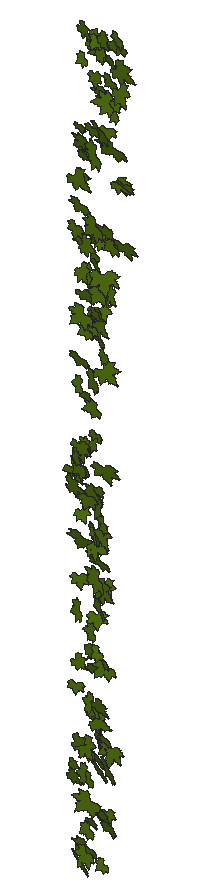
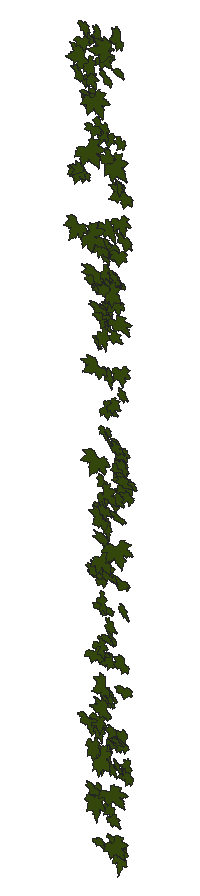
# SketchUp Ruby script. Lengths in inches.
U = 1.inch
M = Sketchup.active_model
def pt(a) = Geom::Point3d.new(a.map { |v| v * U })
def face(e, loops, mat)
  f = e.add_face(loops[0].map { |a| pt(a) })
  loops[1..].each { |l| e.add_face(l.map { |a| pt(a) }).erase! }
  f.material = f.back_material = mat if mat
  f
end
# faces: each face lists its corners as indices into pts; further lists are holes
def faces(e, pts, list, mat = nil) = list.each { |f| face(e, (f[0].is_a?(Array) ? f : [f]).map { |l| l.map { |i| pts[i] } }, mat) }
# xy, xz, yz: faces in a plane at the given z, y or x. An outline is a flat list of corners, or four numbers for a rectangle; further outlines are holes
def ring(l) = l.size == 4 ? [[l[0], l[1]], [l[2], l[1]], [l[2], l[3]], [l[0], l[3]]] : l.each_slice(2).to_a
def flat(e, list, mat, &to3) = list.each { |f| face(e, (f[0].is_a?(Array) ? f : [f]).map { |l| ring(l).map { |u, v| to3.(u, v) } }, mat) }
def xy(e, z, list, mat = nil) = flat(e, list, mat) { |x, y| [x, y, z] }
def xz(e, y, list, mat = nil) = flat(e, list, mat) { |x, z| [x, y, z] }
def yz(e, x, list, mat = nil) = flat(e, list, mat) { |y, z| [x, y, z] }
def lines(e, pts, list) = list.each { |a, b| e.add_line(pt(pts[a]), pt(pts[b])) }
# prism: a flat outline (further loops are holes) pulled along v
def prism(e, loops, v, mat = nil)
  f = face(e, loops, mat); d = Geom::Vector3d.new(v.map { |x| x * U })
  f.pushpull(f.normal.samedirection?(d) ? d.length : -d.length)
end
def box(e, o, s, mat = nil) = prism(e, [[o, [o[0] + s[0], o[1], o[2]], [o[0] + s[0], o[1] + s[1], o[2]], [o[0], o[1] + s[1], o[2]]]], [0, 0, s[2]], mat)
def at(x, y, z, deg = 0) = Geom::Transformation.translation(pt([x, y, z])) * Geom::Transformation.rotation(ORIGIN, Z_AXIS, deg.degrees)
def axes(o, x, y, z) = Geom::Transformation.new([*x, 0, *y, 0, *z, 0, *pt(o).to_a, 1])
def part(name) = M.definitions.add(name)
# library, detail: a bought-in or finely detailed component or shape, given as its bounding box
def library(name, o, s) = part(name).tap { |d| box(d.entities, o, s) }
def detail(e, o, s) = box(e.add_group.entities, o, s)
def put(e, d, t, mat = nil) = e.add_instance(d, t).tap { |i| i.material = mat if mat }
def group(e, t, mat = nil) = e.add_group.tap { |g| g.transformation = t; g.material = mat if mat }.entities
root = M.entities
M.materials.add("[Vegetation Blur 03]").color = [83, 114, 18]
c1 = part("ivy")
xy(c1.entities,0,[[0.782,0,0.786,0,0.787,0.005,0.789,0.009,0.821,0.072,0.875,0.147,1.001,0.272,1.073,0.331,1.137,0.363,1.178,0.379,1.223,0.384,1.272,0.383,1.311,0.374,1.36,0.355,1.399,0.334,1.491,0.285,1.541,0.244,1.583,0.199,1.617,0.15,1.64,0.128,1.662,0.115,1.717,0.105,1.745,0.093,1.784,0.054,1.819,0.057,1.854,0.064,1.882,0.075,1.896,0.074,1.91,0.071,1.937,0.063,1.964,0.053,1.99,0.038,2.016,0.015,2.034,0.002,2.04,0,2.038,0.003,2.036,0.007,2.033,0.038,2.036,0.068,2.045,0.1,2.055,0.116,2.064,0.123,2.077,0.129,2.088,0.129,2.106,0.132,2.118,0.13,2.179,0.132,2.207,0.133,2.225,0.133,2.242,0.138,2.22,0.162,2.207,0.186,2.206,0.213,2.212,0.236,2.228,0.262,2.247,0.274,2.298,0.283,2.355,0.294,2.37,0.296,2.376,0.295,2.377,0.3,2.377,0.303,2.385,0.329,2.411,0.37,2.426,0.392,2.449,0.407,2.511,0.426,2.561,0.444,2.619,0.466,2.589,0.469,2.561,0.476,2.501,0.5,2.449,0.516,2.424,0.523,2.401,0.535,2.377,0.556,2.372,0.568,2.36,0.575,2.268,0.586,2.225,0.592,2.207,0.599,2.194,0.61,2.143,0.65,2.13,0.664,2.122,0.682,2.123,0.7,2.13,0.719,2.148,0.75,2.17,0.781,2.195,0.807,2.221,0.828,2.284,0.874,2.291,0.88,2.288,0.887,2.276,0.9,2.267,0.916,2.265,0.933,2.273,0.967,2.292,1.002,2.313,1.03,2.334,1.054,2.348,1.067,2.358,1.074,2.363,1.076,2.362,1.081,2.35,1.094,2.347,1.11,2.35,1.143,2.359,1.18,2.385,1.254,2.415,1.324,2.448,1.393,2.45,1.4,2.446,1.398,2.44,1.394,2.427,1.383,2.402,1.36,2.376,1.339,2.345,1.324,2.305,1.309,2.282,1.303,2.273,1.306,2.245,1.294,2.212,1.287,2.187,1.291,2.163,1.301,2.142,1.316,2.134,1.327,2.124,1.325,2.09,1.292,2.053,1.259,2.014,1.234,1.973,1.215,1.954,1.21,1.931,1.208,1.909,1.212,1.893,1.22,1.879,1.233,1.872,1.248,1.867,1.281,1.864,1.319,1.821,1.258,1.773,1.197,1.726,1.141,1.698,1.121,1.679,1.116,1.666,1.117,1.647,1.122,1.632,1.129,1.62,1.141,1.617,1.154,1.617,1.219,1.621,1.254,1.623,1.268,1.623,1.281,1.618,1.314,1.606,1.346,1.603,1.375,1.607,1.403,1.603,1.467,1.599,1.499,1.605,1.525,1.614,1.552,1.629,1.577,1.635,1.589,1.629,1.587,1.618,1.582,1.596,1.566,1.581,1.556,1.568,1.552,1.557,1.55,1.545,1.553,1.531,1.562,1.522,1.572,1.504,1.591,1.486,1.611,1.474,1.631,1.457,1.666,1.455,1.684,1.457,1.698,1.452,1.715,1.444,1.728,1.424,1.754,1.419,1.772,1.423,1.786,1.434,1.819,1.444,1.848,1.446,1.855,1.44,1.861,1.43,1.867,1.386,1.904,1.349,1.948,1.326,1.973,1.31,1.995,1.288,2.048,1.284,2.153,1.287,2.254,1.284,2.255,1.282,2.253,1.278,2.247,1.274,2.237,1.266,2.216,1.226,2.125,1.208,2.076,1.184,2.033,1.155,1.984,1.135,1.942,1.111,1.899,1.083,1.861,1.053,1.85,1.059,1.83,1.061,1.809,1.056,1.79,1.049,1.767,1.04,1.749,1.018,1.733,0.994,1.726,0.942,1.734,0.95,1.6875,0.944,1.645,0.932,1.608,0.911,1.585,0.881,1.58,0.854,1.582,0.828,1.588,0.785,1.618,0.773,1.625,0.775,1.614,0.779,1.598,0.796,1.502,0.818,1.402,0.861,1.283,0.882,1.224,0.894,1.174,0.892,1.148,0.886,1.123,0.881,1.107,0.872,1.099,0.849,1.094,0.818,1.092,0.789,1.098,0.762,1.107,0.753,1.113,0.721,1.139,0.698,1.163,0.678,1.194,0.665,1.224,0.628,1.28,0.612,1.312,0.606,1.327,0.606,1.314,0.599,1.282,0.594,1.267,0.581,1.256,0.544,1.245,0.512,1.244,0.473,1.249,0.444,1.256,0.382,1.288,0.339,1.306,0.324,1.316,0.317,1.324,0.309,1.326,0.27,1.314,0.227,1.313,0.185,1.3125,0.152,1.317,0.122,1.328,0.092,1.345,0.073,1.353,0.079,1.338,0.092,1.308,0.117,1.249,0.13,1.215,0.139,1.164,0.147,1.148,0.157,1.136,0.163,1.122,0.174,1.086,0.177,1.067,0.182,1.054,0.186,1.043,0.191,1.038,0.211,1.028,0.237,1.005,0.25,0.974,0.253,0.96,0.25,0.944,0.242,0.914,0.243,0.906,0.249,0.902,0.26,0.894,0.289,0.88,0.307,0.873,0.322,0.862,0.364,0.799,0.403,0.738,0.431,0.709,0.439,0.691,0.441,0.678,0.4375,0.66,0.428,0.645,0.394,0.623,0.303,0.594,0.255,0.581,0.214,0.577,0.179,0.573,0.173,0.568,0.175,0.561,0.167,0.55,0.141,0.523,0.113,0.503,0.077,0.49,0.045,0.486,0.026,0.485,0.019,0.486,0.011,0.483,0,0.471,0.014,0.467,0.044,0.455,0.058,0.447,0.07,0.438,0.097,0.411,0.125,0.394,0.158,0.377,0.174,0.366,0.182,0.359,0.185,0.361,0.242,0.331,0.253,0.316,0.258,0.303,0.262,0.283,0.274,0.278,0.308,0.274,0.341,0.252,0.366,0.226,0.366,0.222,0.37,0.22,0.38,0.221,0.395,0.221,0.425,0.216,0.45,0.207,0.465,0.192,0.473,0.178,0.484,0.15,0.489,0.116,0.483,0.089,0.468,0.058,0.45,0.035,0.435,0.018,0.429,0.011,0.434,0.012,0.438,0.014,0.469,0.019,0.542,0.016,0.581,0.015,0.612,0.027,0.68,0.055,0.696,0.057,0.712,0.052,0.73,0.045,0.741,0.036,0.766,0.014]])
p = [[138.74,174.5,142.56],[138.66,174.5,142.56]]
lines(root,p,[[0,1]])
put(root,c1,axes([134.2,173.7,121.63],[0.07333,0.12212,0.31359],[0.38829,0.01811,-0.06159],[0.01986,-0.80476,0.0462]),"[Vegetation Blur 03]")
put(root,c1,axes([134.3,173.7,106.65],[0.09053,-0.05831,0.23092],[0.28382,-0.01925,-0.07488],[-0.01758,-0.61103,-0.01968]),"[Vegetation Blur 03]")
put(root,c1,axes([134.28,173.7,111.08],[0.35798,0.03491,0.00358],[0.00487,-0.0205,-0.29237],[0.01684,-0.73641,0.00831]),"[Vegetation Blur 03]")
put(root,c1,axes([134.47,173.7,128.12],[0.41941,-0.00434,-0.1684],[-0.2031,0.16133,-0.33757],[-0.03648,-0.94822,-0.05667]),"[Vegetation Blur 03]")
put(root,c1,axes([133.875,173.7,121.9],[0.48195,0.00963,0.21143],[0.25864,0.04977,-0.39304],[0.01557,-1.12486,-0.01558]),"[Vegetation Blur 03]")
put(root,c1,axes([134.5625,173.7,136.09],[0.40291,0.01111,-0.21009],[-0.25613,0.11786,-0.3262],[-0.02632,-0.9768,-0.04175]),"[Vegetation Blur 03]")
put(root,c1,axes([135.08,173.7,126.88],[0.08976,-0.09939,-0.28739],[-0.34963,0.10974,-0.07871],[-0.06393,-0.7397,0.02694]),"[Vegetation Blur 03]")
put(root,c1,axes([135.09,173.7,139.4],[0.2991,0.11532,-0.48246],[-0.59082,0.19391,-0.23668],[-0.05934,-1.34945,-0.07524]),"[Vegetation Blur 03]")
put(root,c1,axes([134.46,173.7,118.99],[0.56725,0.10726,-0.27566],[-0.34171,0.20149,-0.45603],[-0.00596,-1.34353,-0.0904]),"[Vegetation Blur 03]")
put(root,c1,axes([134.92,173.7,115.48],[0.25494,-0.21897,-0.29058],[-0.35433,0.12452,-0.22182],[-0.11199,-0.89248,0.04035]),"[Vegetation Blur 03]")
put(root,c1,axes([134.16,173.7,106.08],[0.21568,-0.13397,0.30172],[0.37321,-0.01782,-0.17894],[-0.04036,-0.88058,-0.04228]),"[Vegetation Blur 03]")
put(root,c1,axes([134.34,173.7,134.82],[0.45457,-0.14322,-0.01986],[-0.02603,-0.01905,-0.37516],[-0.06898,-0.93657,0.01067]),"[Vegetation Blur 03]")
put(root,c1,axes([134.97,173.7,103.27],[0.36107,0.086,-0.36328],[-0.44668,0.11955,-0.29126],[-0.01905,-1.17336,-0.0563]),"[Vegetation Blur 03]")
put(root,c1,axes([134.21,173.7,120.8],[0.10325,-0.14377,0.42811],[0.52829,-0.03594,-0.08677],[-0.03077,-1.09956,-0.05314]),"[Vegetation Blur 03]")
put(root,c1,axes([134.5,173.7,102.52],[0.54071,-0.2448,-0.19934],[-0.20803,0.34691,-0.44288],[-0.17473,-1.17061,-0.08956]),"[Vegetation Blur 03]")
put(root,c1,axes([134.57,173.7,134.13],[0.37713,0.02521,-0.05482],[-0.06814,0.09104,-0.30568],[0.00422,-0.78299,-0.03731]),"[Vegetation Blur 03]")
put(root,c1,axes([134.875,173.7,130.76],[0.44525,-0.05596,-0.30949],[-0.38019,-0.06333,-0.36251],[-0.0007,-1.20185,0.03351]),"[Vegetation Blur 03]")
put(root,c1,axes([135.45,173.7,132.39],[0.11247,0.10768,-0.41349],[-0.50254,0.19726,-0.08297],[-0.08291,-1.04957,-0.05801]),"[Vegetation Blur 03]")
put(root,c1,axes([134.4,173.7,116.58],[0.38704,0.02073,0.09682],[0.11906,-0.06304,-0.31489],[0.00062,-0.83064,0.02631]),"[Vegetation Blur 03]")
put(root,c1,axes([134.79,173.7,123.08],[0.46711,-0.27655,-0.25561],[-0.31156,0.09667,-0.39569],[-0.13813,-1.15324,0.02812]),"[Vegetation Blur 03]")
put(root,c1,axes([134.6,173.7,139.86],[0.29162,-0.09248,0.04712],[0.06325,0.07335,-0.23812],[-0.03677,-0.60733,-0.03593]),"[Vegetation Blur 03]")
put(root,c1,axes([134.36,173.7,111.95],[0.20869,-0.00294,0.30527],[0.37402,-0.00987,-0.17032],[-0.00489,-0.88135,0.00089]),"[Vegetation Blur 03]")
put(root,c1,axes([134.53,173.7,122.5625],[0.11578,-0.07742,0.31422],[0.36947,-0.22297,-0.09932],[-0.11465,-0.79672,-0.00274]),"[Vegetation Blur 03]")
put(root,c1,axes([134.08,173.7,136.79],[0.38841,-0.03974,0.39058],[0.47889,0.01108,-0.31703],[-0.00798,-1.26829,-0.01501]),"[Vegetation Blur 03]")
put(root,c1,axes([134.88,173.7,137.65],[0.29613,-0.07388,-0.10232],[-0.12287,0.05638,-0.24327],[-0.04369,-0.65932,-0.00934]),"[Vegetation Blur 03]")
put(root,c1,axes([135.37,173.7,107.11],[0.14128,-0.20319,-0.29587],[-0.36071,0.14973,-0.1309],[-0.10517,-0.78653,0.05152]),"[Vegetation Blur 03]")
put(root,c1,axes([135.1,173.7,143.71],[0.23115,-0.1069,-0.165],[-0.20647,-0.0259,-0.19002],[-0.03067,-0.63139,0.03573]),"[Vegetation Blur 03]")
put(root,c1,axes([135.41,173.7,126.21],[0.08326,0.10722,-0.24971],[-0.31037,0.02564,-0.0672],[0.00148,-0.65202,-0.0437]),"[Vegetation Blur 03]")
put(root,c1,axes([134.48,173.7,107.61],[0.11289,-0.08937,0.40816],[0.50197,0.01041,-0.09212],[-0.00461,-1.05497,-0.03549]),"[Vegetation Blur 03]")
put(root,c1,axes([135.47,173.7,123.94],[0.13432,-0.12713,-0.31462],[-0.38869,0.03529,-0.11278],[-0.03669,-0.83931,0.04291]),"[Vegetation Blur 03]")
put(root,c1,axes([134.91,173.7,138.74],[0.29319,-0.08212,-0.05398],[-0.06371,0.04494,-0.24127],[-0.04367,-0.61685,-0.01039]),"[Vegetation Blur 03]")
put(root,c1,axes([134.6,173.7,119.81],[0.27283,0.0757,0.1916],[0.23721,-0.13013,-0.2169],[-0.01401,-0.72914,0.0586]),"[Vegetation Blur 03]")
put(root,c1,axes([134.38,173.7,123.48],[0.52424,-0.12738,0.15619],[0.18843,-0.07357,-0.4307],[-0.07036,-1.14606,0.01029]),"[Vegetation Blur 03]")
put(root,c1,axes([135.38,173.7,129.78],[0.19574,-0.01438,-0.25163],[-0.30815,-0.03945,-0.1593],[0.01245,-0.75048,0.0132]),"[Vegetation Blur 03]")
put(root,c1,axes([135.15,173.7,105.83],[0.47968,0.02946,-0.35016],[-0.4281,-0.06549,-0.39149],[0.03188,-1.32271,0.01158]),"[Vegetation Blur 03]")
put(root,c1,axes([135.65,173.7,132.9],[0.09556,-0.13792,-0.34176],[-0.41905,0.10501,-0.08471],[-0.06516,-0.87761,0.04357]),"[Vegetation Blur 03]")
put(root,c1,axes([134.79,173.7,122.375],[0.34163,-0.14558,0.05444],[0.07406,0.06471,-0.28235],[-0.063,-0.71335,-0.03672]),"[Vegetation Blur 03]")
put(root,c1,axes([134.59,173.7,132.14],[0.2559,0.03571,0.2999],[0.36108,-0.20047,-0.20147],[-0.07032,-0.89939,0.05682]),"[Vegetation Blur 03]")
put(root,c1,axes([135.25,173.7,108.26],[0.31122,-0.06083,-0.21678],[-0.26689,-0.02709,-0.25402],[-0.01391,-0.84152,0.02385]),"[Vegetation Blur 03]")
put(root,c1,axes([135.4,173.7,104.21],[0.24157,-0.07416,-0.2538],[-0.31175,0.01688,-0.19842],[-0.02861,-0.81014,0.0191]),"[Vegetation Blur 03]")
put(root,c1,axes([134.6,173.7,131.19],[0.40086,-0.0573,0.17483],[0.21594,0.13183,-0.32299],[0.00594,-0.92596,-0.0568]),"[Vegetation Blur 03]")
put(root,c1,axes([134.9,173.7,138.23],[0.11718,-0.12684,0.22641],[0.28293,-0.00575,-0.09804],[-0.02661,-0.61967,-0.04543]),"[Vegetation Blur 03]")
put(root,c1,axes([134.81,173.7,121.18],[0.52679,-0.06661,-0.07919],[-0.09633,0.02908,-0.43069],[-0.03439,-1.10187,-0.00658]),"[Vegetation Blur 03]")
put(root,c1,axes([135.79,173.7,110.77],[0.05013,-0.17245,-0.31461],[-0.38087,0.18721,-0.05657],[-0.1028,-0.77773,0.05615]),"[Vegetation Blur 03]")
put(root,c1,axes([135,173.7,102.99],[0.48428,-0.17048,-0.13656],[-0.17611,-0.0992,-0.39652],[-0.06201,-1.04969,0.05965]),"[Vegetation Blur 03]")
put(root,c1,axes([135.89,173.7,107.78],[0.15704,0.2136,-0.46973],[-0.57168,0.3147,-0.1048],[-0.12334,-1.18664,-0.11235]),"[Vegetation Blur 03]")
put(root,c1,axes([135.49,173.7,106.8],[0.21308,-0.10262,-0.22404],[-0.27243,0.07685,-0.17812],[-0.0602,-0.71097,0.01308]),"[Vegetation Blur 03]")
put(root,c1,axes([135.8125,173.7,114.47],[0.09612,-0.08439,-0.33414],[-0.40558,0.12635,-0.08273],[-0.06933,-0.85613,0.02072]),"[Vegetation Blur 03]")
put(root,c1,axes([135.82,173.7,121.61],[0.20248,0.05039,-0.42079],[-0.51446,0.11243,-0.16277],[-0.042,-1.13431,-0.03483]),"[Vegetation Blur 03]")
put(root,c1,axes([134.9,173.7,133.32],[0.06821,0.02412,0.38984],[0.47536,-0.1037,-0.05439],[-0.04826,-0.98747,0.01524]),"[Vegetation Blur 03]")
put(root,c1,axes([134.76,173.7,144.75],[0.24867,-0.15858,0.33537],[0.40835,-0.11898,-0.21053],[-0.08971,-0.98119,-0.02867]),"[Vegetation Blur 03]")
put(root,c1,axes([135.82,173.7,125.97],[0.16222,0.03807,-0.33908],[-0.41557,-0.02093,-0.13279],[0.01621,-0.91758,-0.01104]),"[Vegetation Blur 03]")
put(root,c1,axes([134.57,173.7,107.83],[0.38921,-0.01895,0.37093],[0.44943,-0.16908,-0.31546],[-0.06835,-1.21968,0.03797]),"[Vegetation Blur 03]")
put(root,c1,axes([135.86,173.7,133.18],[0.08292,0.05054,-0.29306],[-0.34577,0.22171,-0.05915],[-0.09993,-0.72524,-0.0385]),"[Vegetation Blur 03]")
put(root,c1,axes([135.69,173.7,118.22],[0.33518,0.12814,-0.38098],[-0.46864,0.20726,-0.26366],[-0.04654,-1.16428,-0.08887]),"[Vegetation Blur 03]")
put(root,c1,axes([135.77,173.7,139.36],[0.33503,-0.17484,-0.44401],[-0.53885,0.1655,-0.28108],[-0.11328,-1.30432,0.02385]),"[Vegetation Blur 03]")
put(root,c1,axes([136.19,173.7,121.03],[0.10156,-0.07064,-0.4993],[-0.59327,0.30784,-0.08723],[-0.15326,-1.23847,0.0068]),"[Vegetation Blur 03]")
put(root,c1,axes([135.29,173.7,140.1],[0.37183,-0.05449,-0.06268],[-0.07386,0.08152,-0.30299],[-0.03383,-0.77703,-0.02739]),"[Vegetation Blur 03]")
put(root,c1,axes([135.92,173.7,117.5],[0.29364,-0.08887,-0.43973],[-0.53794,0.07502,-0.24166],[-0.05272,-1.26047,0.01662]),"[Vegetation Blur 03]")
put(root,c1,axes([135.3,173.7,109.67],[0.05383,0.00628,0.24765],[0.29967,-0.10102,-0.04299],[-0.04781,-0.62607,0.00942]),"[Vegetation Blur 03]")
put(root,c1,axes([135.78,173.7,134.52],[0.25146,0.10077,-0.27244],[-0.33679,0.12568,-0.19974],[-0.01997,-0.85077,-0.06178]),"[Vegetation Blur 03]")
put(root,c1,axes([135.6,173.7,135.57],[0.45075,-0.16208,-0.3284],[-0.40131,0.07789,-0.37294],[-0.08406,-1.24093,0.01948]),"[Vegetation Blur 03]")
put(root,c1,axes([135.22,173.7,111.97],[0.19108,-0.09038,0.20852],[0.25839,0.11931,-0.14958],[0.021,-0.6456,-0.05683]),"[Vegetation Blur 03]")
put(root,c1,axes([135.69,173.7,133.79],[0.23501,-0.07019,-0.1629],[-0.19555,0.08472,-0.19365],[-0.05258,-0.62881,-0.00791]),"[Vegetation Blur 03]")
put(root,c1,axes([135.2,173.7,113.14],[0.25479,-0.12423,0.18023],[0.21133,-0.13383,-0.2135],[-0.08804,-0.68079,0.00908]),"[Vegetation Blur 03]")
put(root,c1,axes([135.62,173.7,119.66],[0.37161,-0.21861,-0.25288],[-0.28876,0.23657,-0.31481],[-0.15463,-0.96714,-0.01984]),"[Vegetation Blur 03]")
put(root,c1,axes([135.25,173.7,104.28],[0.2775,-0.12673,0.11481],[0.14869,0.07236,-0.22682],[-0.03837,-0.63611,-0.04867]),"[Vegetation Blur 03]")
put(root,c1,axes([135.95,173.7,144.4],[0.21316,0.03069,-0.31446],[-0.38542,0.04396,-0.17335],[-0.01149,-0.90506,-0.01908]),"[Vegetation Blur 03]")
put(root,c1,axes([135.87,173.7,130.06],[0.16581,-0.12598,-0.20066],[-0.24842,0.03821,-0.1405],[-0.04988,-0.60905,0.03269]),"[Vegetation Blur 03]")
put(root,c1,axes([136.05,173.7,115.84],[0.20676,-0.07941,-0.38547],[-0.44776,0.31453,-0.17016],[-0.15519,-1.01328,-0.02261]),"[Vegetation Blur 03]")
put(root,c1,axes([135.78,173.7,129.8],[0.3273,-0.0909,-0.29956],[-0.34726,0.27044,-0.26563],[-0.12681,-0.97518,-0.04574]),"[Vegetation Blur 03]")
put(root,c1,axes([135.56,173.7,127.63],[0.43303,-0.27941,-0.22313],[-0.26455,0.14367,-0.37028],[-0.1523,-1.044,0.00876]),"[Vegetation Blur 03]")
put(root,c1,axes([135.47,173.7,107.71],[0.5589,-0.19272,-0.25961],[-0.28238,0.39595,-0.45114],[-0.17385,-1.26271,-0.10184]),"[Vegetation Blur 03]")
put(root,c1,axes([135.56,173.7,124.42],[0.33014,-0.06379,-0.05513],[-0.06679,0.02302,-0.2706],[-0.03261,-0.69306,-0.00391]),"[Vegetation Blur 03]")
put(root,c1,axes([135.44,173.7,109.71],[0.13106,0.04715,0.22271],[0.27208,-0.09295,-0.10355],[-0.03102,-0.61597,0.03267]),"[Vegetation Blur 03]")
put(root,c1,axes([135.42,173.7,130.65],[0.34203,-0.05341,0.04309],[0.05121,-0.04542,-0.27956],[-0.02898,-0.71072,0.01463]),"[Vegetation Blur 03]")
put(root,c1,axes([135.64,173.7,144.8125],[0.33694,0.0048,-0.1079],[-0.13035,-0.11296,-0.27192],[0.0222,-0.7362,0.04102]),"[Vegetation Blur 03]")
put(root,c1,axes([135.44,173.7,123.48],[0.09035,0.0602,0.28294],[0.33236,-0.23291,-0.06289],[-0.10289,-0.69949,0.04529]),"[Vegetation Blur 03]")
put(root,c1,axes([135.89,173.7,113.49],[0.26178,-0.07777,-0.19292],[-0.23918,-0.11506,-0.20887],[0.01,-0.71663,0.05447]),"[Vegetation Blur 03]")
put(root,c1,axes([135.35,173.7,114.91],[0.41222,0.08825,0.09854],[0.12607,-0.1297,-0.333],[0.02291,-0.87434,0.05934]),"[Vegetation Blur 03]")
put(root,c1,axes([135.25,173.7,117.91],[0.09143,0.21564,0.47102],[0.58317,-0.16267,-0.06368],[-0.06308,-1.19139,0.09395]),"[Vegetation Blur 03]")
put(root,c1,axes([135.94,173.7,113.27],[0.3587,-0.08547,-0.26789],[-0.31864,0.17898,-0.29317],[-0.08908,-0.98439,-0.03004]),"[Vegetation Blur 03]")
put(root,c1,axes([135.69,173.7,132.04],[0.46854,-0.05722,-0.15501],[-0.19159,-0.07548,-0.38134],[-0.0119,-1.03762,0.03629]),"[Vegetation Blur 03]")
put(root,c1,axes([136.02,173.7,108.8],[0.31159,-0.10577,-0.25159],[-0.29051,0.23223,-0.255],[-0.11522,-0.87155,-0.03742]),"[Vegetation Blur 03]")
put(root,c1,axes([135.44,173.7,142.8],[0.3823,-0.12513,0.1329],[0.15394,-0.13225,-0.31454],[-0.08072,-0.8448,0.02956]),"[Vegetation Blur 03]")
put(root,c1,axes([135.24,173.7,143.86],[0.15219,-0.0035,0.49259],[0.60198,0.09401,-0.12377],[0.04388,-1.27745,-0.01046]),"[Vegetation Blur 03]")
put(root,c1,axes([135.59,173.7,130.125],[0.08947,-0.09548,0.30203],[0.3696,-0.08246,-0.07703],[-0.05008,-0.77914,-0.02886]),"[Vegetation Blur 03]")
put(root,c1,axes([135.98,173.7,142.33],[0.49914,0.06889,-0.35402],[-0.43405,0.1716,-0.40237],[-0.0297,-1.34994,-0.06922]),"[Vegetation Blur 03]")
put(root,c1,axes([136.62,173.7,135.19],[0.20681,0.14961,-0.50522],[-0.62308,0.08477,-0.16594],[-0.01632,-1.34039,-0.06689]),"[Vegetation Blur 03]")
put(root,c1,axes([135.7,173.7,121.4],[0.23912,-0.07387,0.13682],[0.16931,0.00875,-0.19635],[-0.02693,-0.60087,-0.01968]),"[Vegetation Blur 03]")
put(root,c1,axes([135.46,173.7,108.95],[0.10403,0.04174,0.45584],[0.55849,-0.05312,-0.08413],[-0.02168,-1.16792,0.02012]),"[Vegetation Blur 03]")
put(root,c1,axes([136.01,173.7,112.82],[0.41939,0.05909,-0.24373],[-0.29711,-0.06483,-0.343],[0.04165,-1.05748,0.00741]),"[Vegetation Blur 03]")
put(root,c1,axes([135.6875,173.7,133.9],[0.15956,0.10306,0.24419],[0.30313,-0.02658,-0.13017],[0.01203,-0.69728,0.04105]),"[Vegetation Blur 03]")
put(root,c1,axes([135.6,173.7,140.42],[0.59182,-0.28218,-0.07799],[-0.07654,0.18572,-0.49252],[-0.14859,-1.21956,-0.05695]),"[Vegetation Blur 03]")
put(root,c1,axes([136.18,173.7,102.625],[0.26116,-0.07939,-0.16142],[-0.20062,-0.0401,-0.21311],[-0.01886,-0.67295,0.03174]),"[Vegetation Blur 03]")
put(root,c1,axes([135.9,173.7,109.1875],[0.45644,-0.12973,-0.15733],[-0.18474,0.13729,-0.3748],[-0.08372,-1.01031,-0.03073]),"[Vegetation Blur 03]")
put(root,c1,axes([135.61,173.7,130.54],[0.32504,0.10399,0.20827],[0.26014,-0.12611,-0.26052],[0.00118,-0.84097,0.06482]),"[Vegetation Blur 03]")
put(root,c1,axes([136.35,173.7,139.73],[0.44413,0.17265,-0.41061],[-0.51006,0.15289,-0.35736],[-0.00095,-1.3725,-0.09146]),"[Vegetation Blur 03]")
put(root,c1,axes([135.96,173.7,105.05],[0.5663,-0.16171,-0.26651],[-0.30497,0.30432,-0.46069],[-0.14072,-1.31032,-0.0741]),"[Vegetation Blur 03]")
put(root,c1,axes([136.1875,173.7,120.29],[0.32555,-0.21056,-0.17248],[-0.21105,0.06347,-0.27751],[-0.10292,-0.79617,0.02349]),"[Vegetation Blur 03]")
put(root,c1,axes([135.5,173.7,110.29],[0.35259,-0.1904,0.31199],[0.38853,0.00444,-0.29204],[-0.06112,-1.07015,-0.05672]),"[Vegetation Blur 03]")
put(root,c1,axes([136.82,173.7,142.18],[0.12519,-0.10736,-0.42184],[-0.51949,-0.03465,-0.1013],[0.00417,-1.09384,0.04461]),"[Vegetation Blur 03]")
put(root,c1,axes([135.81,173.7,143.92],[0.26564,-0.06538,0.20861],[0.24422,-0.17627,-0.21582],[-0.08188,-0.73784,0.03307]),"[Vegetation Blur 03]")
put(root,c1,axes([135.4,173.7,132.52],[0.63449,0.08244,0.15008],[0.18708,-0.13099,-0.51549],[0.02055,-1.35306,0.05905]),"[Vegetation Blur 03]")
put(root,c1,axes([136.7,173.7,143.91],[0.1485,0.06744,-0.32773],[-0.39216,0.22625,-0.11103],[-0.09244,-0.8515,-0.05546]),"[Vegetation Blur 03]")
put(root,c1,axes([135.59,173.7,129.63],[0.21618,-0.06557,0.43271],[0.52184,-0.19331,-0.17826],[-0.09899,-1.16227,0.00524]),"[Vegetation Blur 03]")
put(root,c1,axes([135.5,173.7,122.7],[0.61927,-0.03223,0.11526],[0.14207,0.12094,-0.50313],[-0.00213,-1.30144,-0.04961]),"[Vegetation Blur 03]")
put(root,c1,axes([135.4,173.7,119.15],[0.45704,-0.07073,0.34791],[0.42202,-0.13355,-0.37354],[-0.06933,-1.27915,0.01976]),"[Vegetation Blur 03]")
put(root,c1,axes([136.24,173.7,107.85],[0.48214,-0.22782,-0.28181],[-0.31501,0.32234,-0.39997],[-0.17959,-1.177,-0.05499]),"[Vegetation Blur 03]")
put(root,c1,axes([135.9375,173.7,104.6875],[0.21432,-0.13844,0.2244],[0.28013,0.00181,-0.17803],[-0.04065,-0.71738,-0.04375]),"[Vegetation Blur 03]")
put(root,c1,axes([135.56,173.7,127.27],[0.38223,0.09975,0.36551],[0.44923,0.00523,-0.31313],[0.03341,-1.2116,0.02874]),"[Vegetation Blur 03]")
put(root,c1,axes([136.18,173.7,128.8125],[0.32645,-0.19251,-0.02516],[-0.03795,-0.04316,-0.27603],[-0.0909,-0.67338,0.02489]),"[Vegetation Blur 03]")
put(root,c1,axes([136.0625,173.7,140.17],[0.36239,0.03439,0.0325],[0.04011,-0.01114,-0.29602],[0.01602,-0.75014,0.00588]),"[Vegetation Blur 03]")
put(root,c1,axes([136.5,173.7,143.07],[0.31224,-0.04153,-0.22289],[-0.2695,0.10455,-0.25454],[-0.04857,-0.84719,-0.02048]),"[Vegetation Blur 03]")
put(root,c1,axes([135.72,173.7,115.93],[0.19345,-0.03327,0.47278],[0.57353,-0.16922,-0.15818],[-0.0831,-1.24533,0.00886]),"[Vegetation Blur 03]")
put(root,c1,axes([135.92,173.7,144.58],[0.22749,-0.09368,0.31124],[0.37139,-0.17878,-0.18927],[-0.09787,-0.89612,0.00522]),"[Vegetation Blur 03]")
put(root,c1,axes([135.9,173.7,116.41],[0.30062,0.06409,0.25513],[0.31279,-0.14376,-0.23982],[-0.02918,-0.88082,0.05771]),"[Vegetation Blur 03]")
put(root,c1,axes([136.76,173.7,134.62],[0.2286,-0.00259,-0.27195],[-0.33307,0.02295,-0.18652],[-0.00991,-0.83122,-0.0043]),"[Vegetation Blur 03]")
put(root,c1,axes([136.11,173.7,104.98],[0.33883,-0.03876,0.14234],[0.17237,-0.07132,-0.27636],[-0.03256,-0.78094,0.01817]),"[Vegetation Blur 03]")
put(root,c1,axes([137.19,173.7,141.72],[0.11758,-0.14394,-0.33997],[-0.41694,0.10295,-0.1029],[-0.06765,-0.88473,0.04334]),"[Vegetation Blur 03]")
put(root,c1,axes([136.32,173.7,141.8],[0.42779,-0.01722,0.00276],[0.0027,-0.07154,-0.34805],[-0.00862,-0.87743,0.02832]),"[Vegetation Blur 03]")
put(root,c1,axes([136.2,173.7,131.4],[0.18898,0.02634,0.37085],[0.44381,-0.22984,-0.14807],[-0.09838,-0.98629,0.04441]),"[Vegetation Blur 03]")
put(root,c1,axes([136.14,173.7,108.68],[0.62343,-0.11777,0.0104],[0.0079,-0.1089,-0.50918],[-0.0581,-1.27854,0.04241]),"[Vegetation Blur 03]")
put(root,c1,axes([136.49,173.7,144.62],[0.24814,-0.07421,0.13501],[0.16554,-0.02052,-0.20443],[-0.03556,-0.61336,-0.0095]),"[Vegetation Blur 03]")
put(root,c1,axes([136.84,173.7,144.75],[0.32819,0.01887,-0.10221],[-0.12554,0.06541,-0.2666],[-0.0028,-0.71988,-0.0269]),"[Vegetation Blur 03]")
put(root,c1,axes([136.91,173.7,145.43],[0.36865,-0.17556,-0.1237],[-0.14943,0.05438,-0.30876],[-0.08901,-0.81841,0.00602]),"[Vegetation Blur 03]")
put(root,c1,axes([136.61,173.7,137.29],[0.29759,0.01634,0.29239],[0.3571,0.0663,-0.24267],[0.02985,-0.95609,-0.01183]),"[Vegetation Blur 03]")
put(root,c1,axes([136.92,173.7,137.7],[0.43208,-0.00485,-0.01137],[-0.01346,0.125,-0.34915],[-0.00429,-0.88078,-0.04949]),"[Vegetation Blur 03]")
put(root,c1,axes([136.71,173.7,142.17],[0.38148,-0.02964,0.33346],[0.3977,-0.23961,-0.3064],[-0.09475,-1.12505,0.05647]),"[Vegetation Blur 03]")
put(root,c1,axes([136.8125,173.7,134.58],[0.54527,-0.10858,0.11727],[0.14945,0.14116,-0.4423],[-0.03309,-1.15173,-0.06527]),"[Vegetation Blur 03]")
put(root,c1,axes([136.65,173.7,143.01],[0.28018,-0.09633,0.48866],[0.59963,-0.03141,-0.22997],[-0.03369,-1.35996,-0.0293]),"[Vegetation Blur 03]")
